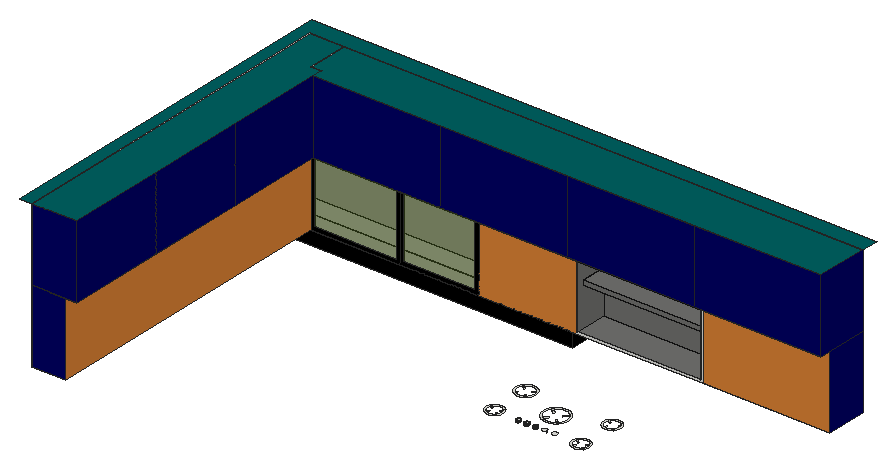
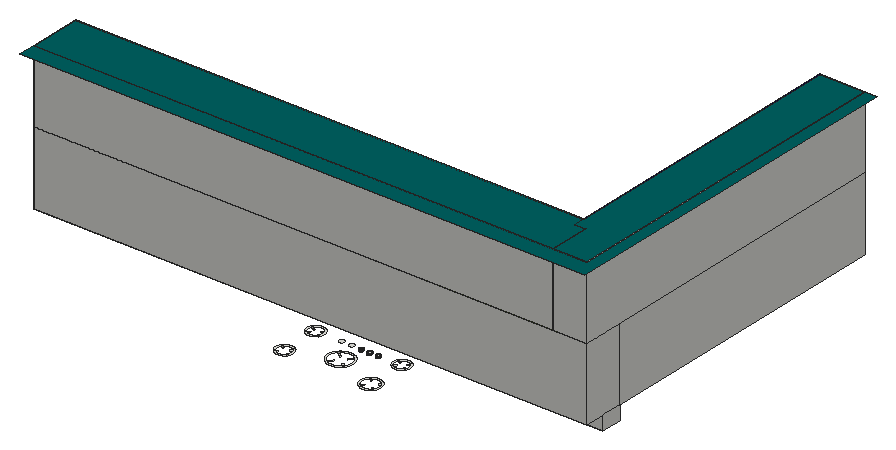
# SketchUp Ruby script. Lengths in inches.
U = 1.inch
M = Sketchup.active_model
def pt(a) = Geom::Point3d.new(a.map { |v| v * U })
def face(e, loops, mat)
  f = e.add_face(loops[0].map { |a| pt(a) })
  loops[1..].each { |l| e.add_face(l.map { |a| pt(a) }).erase! }
  f.material = f.back_material = mat if mat
  f
end
# faces: each face lists its corners as indices into pts; further lists are holes
def faces(e, pts, list, mat = nil) = list.each { |f| face(e, (f[0].is_a?(Array) ? f : [f]).map { |l| l.map { |i| pts[i] } }, mat) }
# xy, xz, yz: faces in a plane at the given z, y or x. An outline is a flat list of corners, or four numbers for a rectangle; further outlines are holes
def ring(l) = l.size == 4 ? [[l[0], l[1]], [l[2], l[1]], [l[2], l[3]], [l[0], l[3]]] : l.each_slice(2).to_a
def flat(e, list, mat, &to3) = list.each { |f| face(e, (f[0].is_a?(Array) ? f : [f]).map { |l| ring(l).map { |u, v| to3.(u, v) } }, mat) }
def xy(e, z, list, mat = nil) = flat(e, list, mat) { |x, y| [x, y, z] }
def xz(e, y, list, mat = nil) = flat(e, list, mat) { |x, z| [x, y, z] }
def yz(e, x, list, mat = nil) = flat(e, list, mat) { |y, z| [x, y, z] }
def lines(e, pts, list) = list.each { |a, b| e.add_line(pt(pts[a]), pt(pts[b])) }
# prism: a flat outline (further loops are holes) pulled along v
def prism(e, loops, v, mat = nil)
  f = face(e, loops, mat); d = Geom::Vector3d.new(v.map { |x| x * U })
  f.pushpull(f.normal.samedirection?(d) ? d.length : -d.length)
end
def box(e, o, s, mat = nil) = prism(e, [[o, [o[0] + s[0], o[1], o[2]], [o[0] + s[0], o[1] + s[1], o[2]], [o[0], o[1] + s[1], o[2]]]], [0, 0, s[2]], mat)
def at(x, y, z, deg = 0) = Geom::Transformation.translation(pt([x, y, z])) * Geom::Transformation.rotation(ORIGIN, Z_AXIS, deg.degrees)
def axes(o, x, y, z) = Geom::Transformation.new([*x, 0, *y, 0, *z, 0, *pt(o).to_a, 1])
def part(name) = M.definitions.add(name)
# library, detail: a bought-in or finely detailed component or shape, given as its bounding box
def library(name, o, s) = part(name).tap { |d| box(d.entities, o, s) }
def detail(e, o, s) = box(e.add_group.entities, o, s)
def put(e, d, t, mat = nil) = e.add_instance(d, t).tap { |i| i.material = mat if mat }
def group(e, t, mat = nil) = e.add_group.tap { |g| g.transformation = t; g.material = mat if mat }.entities
root = M.entities
M.materials.add("[0079_Teal]").color = [0, 96, 96]
M.materials.add("[0105_Navy]").color = [0, 0, 99]
M.materials.add("[Color M09]").color = [0, 0, 0]
M.materials.add("[Translucent Glass Dark Green]").color = [50, 73, 4]
M.materials["[Translucent Glass Dark Green]"].alpha = 0.5
M.materials.add("[Translucent Glass Gray]").color = [0, 0, 0]
M.materials["[Translucent Glass Gray]"].alpha = 0.5
M.materials.add("[Wood Bamboo]").color = [219, 130, 53]
xy(root,254.3125,[[832.58,637.12,838.75,642.52,837.78,643.6,831.63,638.07],[859.45,639.53,860.47,641.1,853.45,645.15,852.51,643.53],[834.88,653.71,835.82,655.33,829.43,659.02,828.58,657.35],[852.77,654.76,859.45,660.59,858.27,662.05,851.61,656.05]])
xy(root,254.5,[[834.42,730.4,838.85,735.32,837.46,736.57,832.96,731.58],[858.27,732.91,859.45,734.36,854.32,738.09,853.22,736.57],[833.38,750.99,834.48,752.51,830.45,755.43,829.43,753.86],[854.32,752.51,858.27,756.89,856.94,758.22,852.93,753.76]])
xy(root,255.0625,[[722.22,684.24,731.81,694.89,729.65,696.84,720.06,686.1875,721.09,685.16],[758.29,685.16,760.34,687.22,749.23,697.28,747.14,694.89],[726.2,714.05,728.12,716.18,719.03,724.42,717.2,722.15],[749.23,714.24,759.31,725.44,758.29,726.47,757.16,727.39,757.05,727.28,747.07,716.18]])
xy(root,255.1875,[[647.3,727.57,649.04,728.98,643.57,734.45,641.99,732.875],[619.69,729.66,619.86,729.83,624.69,733.98,623.16,735.77,618.09,731.4375,618.79,730.5625],[645.15,751.5625,652.04,757.49,650.63,759.23,643.67,753.28],[623.16,751.71,624.74,753.28,618.79,759.23,617.38,757.49]])
xy(root,255.75,[[622.85,637.29,629.08,642.73,627.88,644.1,621.58,638.6],[649.15,640.36,649.66,641.12,650.09,641.92,643.42,645.67,642.53,644.09],[624.89,654.02,625.78,655.61,619.76,659,618.91,657.39],[642.65,654.57,648.96,660.08,647.84,661.51,641.46,655.95]])
xy(root,256.875,[[[844.95,629.31,847.12,629.42,849.27,629.76,851.36,630.32,853.39,631.1,855.33,632.09,857.15,633.27,858.84,634.64,860.37,636.17,861.74,637.86,862.92,639.68,863.91,641.62,864.6875,643.65,865.25,645.74,865.59,647.89,865.7,650.06,865.59,652.23,865.25,654.375,864.6875,656.47,863.91,658.5,862.92,660.43,861.74,662.26,860.37,663.94,858.84,665.48,857.15,666.85,855.33,668.03,853.39,669.02,851.36,669.79,849.27,670.36,847.12,670.7,844.95,670.81,842.78,670.7,840.64,670.36,838.54,669.79,836.51,669.02,834.58,668.03,832.76,666.85,831.07,665.48,829.53,663.94,828.16,662.26,826.98,660.43,826,658.5,825.22,656.47,824.66,654.375,824.32,652.23,824.2,650.06,824.32,647.89,824.66,645.74,825.22,643.65,826,641.62,826.98,639.68,828.16,637.86,829.53,636.17,831.07,634.64,832.76,633.27,834.58,632.09,836.51,631.1,838.54,630.32,840.64,629.76,842.78,629.42],[844.95,632.14,843.08,632.24,841.23,632.53,839.41,633.01,837.66,633.6875,835.99,634.54,834.42,635.56,832.96,636.74,831.63,638.07,830.45,639.53,829.43,641.1,828.58,642.77,827.91,644.52,827.42,646.33,827.13,648.1875,827.03,650.06,827.13,651.93,827.42,653.79,827.91,655.6,828.58,657.35,829.43,659.02,830.45,660.59,831.63,662.05,832.96,663.38,834.42,664.56,835.99,665.58,837.66,666.43,839.41,667.1,841.23,667.59,843.08,667.88,844.95,667.98,846.82,667.88,848.68,667.59,850.49,667.1,852.24,666.43,853.91,665.58,855.49,664.56,856.94,663.38,858.27,662.05,859.45,660.59,860.47,659.02,861.32,657.35,862,655.6,862.48,653.79,862.77,651.93,862.875,650.06,862.77,648.1875,862.48,646.33,862,644.52,861.32,642.77,860.47,641.1,859.45,639.53,858.27,638.07,856.94,636.74,855.49,635.56,853.91,634.54,852.24,633.6875,850.49,633.01,848.68,632.53,846.82,632.24]],[[634.4,629.8125,636.51,629.89,638.61,630.1875,640.67,630.71,642.66,631.43,644.5625,632.37,646.36,633.49,648.02,634.8,649.55,636.28,650.91,637.9,652.09,639.66,653.08,641.54,653.87,643.5,654.45,645.54,654.8125,647.63,654.96,649.74,654.88,651.86,654.58,653.96,654.0625,656.02,653.33,658.01,652.4,659.91,651.28,661.71,649.97,663.375,648.49,664.9,646.87,666.25,645.11,667.4375,643.23,668.43,641.27,669.22,639.23,669.8,637.14,670.16,635.02,670.31,632.91,670.23,630.81,669.93,628.75,669.41,626.76,668.68,624.86,667.75,623.0625,666.625,621.4,665.32,619.875,663.84,618.51,662.21,617.33,660.45,616.34,658.58,615.55,656.61,614.97,654.58,614.61,652.49,614.46,650.375,614.54,648.26,614.84,646.16,615.36,644.1,616.08,642.11,617.02,640.21,618.14,638.41,619.45,636.74,620.93,635.22,622.55,633.86,624.3125,632.68,626.1875,631.69,628.15,630.9,630.19,630.32,632.28,629.96],[634.4375,632.64,632.62,632.76,630.82,633.08,629.07,633.58,627.38,634.26,625.77,635.11,624.25,636.125,622.85,637.29,621.58,638.6,620.46,640.04,619.49,641.58,618.6875,643.22,618.06,644.93,617.61,646.7,617.36,648.51,617.29,650.33,617.41,652.15,617.73,653.95,618.23,655.7,618.91,657.39,619.76,659,620.78,660.52,621.95,661.92,623.25,663.19,624.69,664.31,626.23,665.28,627.87,666.08,629.58,666.71,631.35,667.15,633.16,667.41,634.98,667.48,636.8,667.35,638.6,667.04,640.35,666.54,642.04,665.86,643.65,665.01,645.17,663.99,646.57,662.82,647.84,661.51,648.96,660.08,649.93,658.53,650.73,656.9,651.36,655.18,651.8,653.42,652.0625,651.61,652.13,649.79,652.01,647.97,651.69,646.17,651.19,644.42,650.51,642.73,649.66,641.12,648.64,639.6,647.47,638.2,646.16,636.93,644.73,635.81,643.19,634.84,641.55,634.04,639.84,633.41,638.07,632.96,636.26,632.71]],[713.34,644.32,713.91,644.35,714.47,644.4375,715.02,644.58,715.55,644.79,716.06,645.05,716.53,645.36,716.98,645.71,717.38,646.12,717.74,646.56,718.05,647.04,718.31,647.54,718.51,648.07,718.66,648.625,718.75,649.1875,718.78,649.75,718.75,650.32,718.66,650.89,718.51,651.43,718.31,651.97,718.05,652.47,717.74,652.95,717.38,653.39,716.98,653.8,716.53,654.15,716.06,654.46,715.55,654.72,715.02,654.93,714.47,655.07,713.91,655.16,713.34,655.19,712.77,655.16,712.21,655.07,711.66,654.93,711.125,654.72,710.62,654.46,710.14,654.15,709.7,653.8,709.3,653.39,708.9375,652.95,708.63,652.47,708.37,651.97,708.17,651.43,708.02,650.89,707.93,650.32,707.9,649.75,707.93,649.1875,708.02,648.625,708.17,648.07,708.37,647.54,708.63,647.04,708.9375,646.56,709.3,646.12,709.7,645.71,710.14,645.36,710.62,645.05,711.125,644.79,711.66,644.58,712.21,644.4375,712.77,644.35],[781.2,644.44,781.76,644.47,782.31,644.56,782.85,644.7,783.36,644.9,783.86,645.15,784.33,645.46,784.76,645.81,785.15,646.2,785.5,646.63,785.8,647.1,786.06,647.59,786.26,648.11,786.4,648.65,786.49,649.2,786.52,649.75,786.49,650.31,786.4,650.86,786.26,651.4,786.06,651.92,785.8,652.41,785.5,652.88,785.15,653.31,784.76,653.7,784.33,654.05,783.86,654.36,783.36,654.61,782.85,654.81,782.31,654.95,781.76,655.04,781.2,655.07,780.65,655.04,780.1,654.95,779.5625,654.81,779.04,654.61,778.55,654.36,778.08,654.05,777.65,653.7,777.26,653.31,776.91,652.88,776.6,652.41,776.35,651.92,776.15,651.4,776.01,650.86,775.92,650.31,775.89,649.75,775.92,649.2,776.01,648.65,776.15,648.11,776.35,647.59,776.6,647.1,776.91,646.63,777.26,646.2,777.65,645.81,778.08,645.46,778.55,645.15,779.04,644.9,779.5625,644.7,780.1,644.56,780.65,644.47],[756.84,644.69,757.37,644.72,757.89,644.8,758.4,644.94,758.9,645.13,759.37,645.37,759.82,645.66,760.23,645.99,760.6,646.37,760.94,646.78,761.22,647.22,761.46,647.7,761.65,648.19,761.79,648.7,761.875,649.23,761.9,649.75,761.875,650.28,761.79,650.81,761.65,651.32,761.46,651.8125,761.22,652.29,760.94,652.73,760.6,653.14,760.23,653.52,759.82,653.85,759.37,654.14,758.9,654.38,758.4,654.57,757.89,654.71,757.37,654.79,756.84,654.82,756.3125,654.79,755.79,654.71,755.28,654.57,754.78,654.38,754.31,654.14,753.86,653.85,753.45,653.52,753.08,653.14,752.74,652.73,752.46,652.29,752.21,651.8125,752.02,651.32,751.89,650.81,751.8,650.28,751.78,649.75,751.8,649.23,751.89,648.7,752.02,648.19,752.21,647.7,752.46,647.22,752.74,646.78,753.08,646.37,753.45,645.99,753.86,645.66,754.31,645.37,754.78,645.13,755.28,644.94,755.79,644.8,756.3125,644.72],
  [734.71,644.78,735.23,644.81,735.75,644.89,736.25,645.03,736.74,645.21,737.2,645.45,737.64,645.73,738.04,646.06,738.41,646.43,738.74,646.83,739.02,647.27,739.26,647.73,739.44,648.22,739.58,648.72,739.66,649.23,739.6875,649.75,739.66,650.27,739.58,650.79,739.44,651.29,739.26,651.78,739.02,652.24,738.74,652.68,738.41,653.08,738.04,653.45,737.64,653.78,737.2,654.0625,736.74,654.3,736.25,654.48,735.75,654.62,735.23,654.7,734.71,654.73,734.19,654.7,733.68,654.62,733.18,654.48,732.69,654.3,732.23,654.0625,731.79,653.78,731.39,653.45,731.02,653.08,730.69,652.68,730.41,652.24,730.17,651.78,729.98,651.29,729.85,650.79,729.77,650.27,729.74,649.75,729.77,649.23,729.85,648.72,729.98,648.22,730.17,647.73,730.41,647.27,730.69,646.83,731.02,646.43,731.39,646.06,731.79,645.73,732.23,645.45,732.69,645.21,733.18,645.03,733.68,644.89,734.19,644.81],[693.15,644.94,693.65,644.97,694.15,645.05,694.63,645.18,695.1,645.36,695.55,645.59,695.97,645.86,696.37,646.18,696.72,646.53,697.04,646.93,697.3125,647.35,697.54,647.8,697.72,648.27,697.85,648.75,697.93,649.25,697.96,649.75,697.93,650.26,697.85,650.76,697.72,651.24,697.54,651.71,697.3125,652.16,697.04,652.58,696.72,652.97,696.37,653.33,695.97,653.65,695.55,653.92,695.1,654.15,694.63,654.33,694.15,654.46,693.65,654.54,693.15,654.57,692.64,654.54,692.14,654.46,691.66,654.33,691.1875,654.15,690.74,653.92,690.32,653.65,689.93,653.33,689.57,652.97,689.25,652.58,688.98,652.16,688.75,651.71,688.57,651.24,688.4375,650.76,688.36,650.26,688.33,649.75,688.36,649.25,688.4375,648.75,688.57,648.27,688.75,647.8,688.98,647.35,689.25,646.93,689.57,646.53,689.93,646.18,690.32,645.86,690.74,645.59,691.1875,645.36,691.66,645.18,692.14,645.05,692.64,644.97],[[739.6875,675.19,742.89,675.36,746.05,675.86,749.15,676.69,752.14,677.84,755,679.29,757.6875,681.04,760.18,683.06,762.45,685.32,764.46,687.82,766.21,690.5,767.66,693.36,768.8125,696.35,769.64,699.45,770.14,702.61,770.3125,705.82,770.14,709.02,769.64,712.18,768.8125,715.28,767.66,718.27,766.21,721.13,764.46,723.82,762.45,726.31,760.18,728.57,757.6875,730.59,755,732.34,752.14,733.79,749.15,734.94,746.05,735.77,742.89,736.27,739.6875,736.44,736.49,736.27,733.32,735.77,730.22,734.94,727.23,733.79,724.375,732.34,721.6875,730.59,719.19,728.57,716.93,726.31,714.91,723.82,713.16,721.13,711.71,718.27,710.5625,715.28,709.73,712.18,709.23,709.02,709.0625,705.82,709.23,702.61,709.73,699.45,710.5625,696.35,711.71,693.36,713.16,690.5,714.91,687.82,716.93,685.32,719.19,683.06,721.6875,681.04,724.375,679.29,727.23,677.84,730.22,676.69,733.32,675.86,736.49,675.36],[739.6875,678.02,736.78,678.17,733.91,678.625,731.1,679.38,728.38,680.42,725.79,681.74,723.35,683.33,721.09,685.16,719.03,687.22,717.2,689.48,715.61,691.92,714.29,694.51,713.25,697.23,712.5,700.04,712.04,702.91,711.89,705.82,712.04,708.72,712.5,711.6,713.25,714.41,714.29,717.12,715.61,719.71,717.2,722.15,719.03,724.42,721.09,726.47,723.35,728.3,725.79,729.89,728.38,731.21,731.1,732.25,733.91,733,736.78,733.46,739.6875,733.61,742.59,733.46,745.47,733,748.28,732.25,750.99,731.21,753.58,729.89,756.03,728.3,758.29,726.47,760.34,724.42,762.17,722.15,763.76,719.71,765.08,717.12,766.12,714.41,766.875,711.6,767.33,708.72,767.48,705.82,767.33,702.91,766.875,700.04,766.12,697.23,765.08,694.51,763.76,691.92,762.17,689.48,760.34,687.22,758.29,685.16,756.03,683.33,753.58,681.74,750.99,680.42,748.28,679.38,745.47,678.625,742.59,678.17]],[[634.71,720.65,637.24,720.78,639.75,721.18,642.2,721.84,644.57,722.74,646.83,723.9,648.96,725.28,650.9375,726.875,652.73,728.67,654.33,730.64,655.71,732.77,656.86,735.03,657.77,737.4,658.43,739.86,658.83,742.36,658.96,744.9,658.83,747.43,658.43,749.94,657.77,752.39,656.86,754.76,655.71,757.02,654.33,759.15,652.73,761.125,650.9375,762.92,648.96,764.52,646.83,765.9,644.57,767.05,642.2,767.96,639.75,768.62,637.24,769.02,634.71,769.15,632.18,769.02,629.67,768.62,627.22,767.96,624.85,767.05,622.58,765.9,620.46,764.52,618.48,762.92,616.6875,761.125,615.09,759.15,613.71,757.02,612.56,754.76,611.65,752.39,610.99,749.94,610.59,747.43,610.46,744.9,610.59,742.36,610.99,739.86,611.65,737.4,612.56,735.03,613.71,732.77,615.09,730.64,616.6875,728.67,618.48,726.875,620.46,725.28,622.58,723.9,624.85,722.74,627.22,721.84,629.67,721.18,632.18,720.78],[634.71,723.48,632.47,723.59,630.26,723.94,628.09,724.53,626,725.33,624,726.35,622.12,727.57,620.375,728.98,618.79,730.5625,617.38,732.31,616.16,734.1875,615.14,736.19,614.34,738.28,613.76,740.44,613.41,742.66,613.29,744.9,613.41,747.14,613.76,749.35,614.34,751.52,615.14,753.61,616.16,755.61,617.38,757.49,618.79,759.23,620.375,760.82,622.12,762.23,624,763.45,626,764.47,628.09,765.27,630.26,765.85,632.47,766.2,634.71,766.32,636.95,766.2,639.16,765.85,641.33,765.27,643.42,764.47,645.42,763.45,647.3,762.23,649.04,760.82,650.63,759.23,652.04,757.49,653.26,755.61,654.28,753.61,655.08,751.52,655.66,749.35,656.01,747.14,656.13,744.9,656.01,742.66,655.66,740.44,655.08,738.28,654.28,736.19,653.26,734.1875,652.04,732.31,650.63,730.5625,649.04,728.98,647.3,727.57,645.42,726.35,643.42,725.33,641.33,724.53,639.16,723.94,636.95,723.59]],[[844.95,724.15,847.12,724.26,849.27,724.6,851.36,725.16,853.39,725.94,855.33,726.93,857.15,728.11,858.84,729.48,860.37,731.01,861.74,732.7,862.92,734.52,863.91,736.46,864.6875,738.49,865.25,740.58,865.59,742.73,865.7,744.9,865.59,747.07,865.25,749.21,864.6875,751.31,863.91,753.34,862.92,755.27,861.74,757.09,860.37,758.78,858.84,760.32,857.15,761.69,855.33,762.87,853.39,763.85,851.36,764.63,849.27,765.19,847.12,765.53,844.95,765.65,842.78,765.53,840.64,765.19,838.54,764.63,836.51,763.85,834.58,762.87,832.76,761.69,831.07,760.32,829.53,758.78,828.16,757.09,826.98,755.27,826,753.34,825.22,751.31,824.66,749.21,824.32,747.07,824.2,744.9,824.32,742.73,824.66,740.58,825.22,738.49,826,736.46,826.98,734.52,828.16,732.7,829.53,731.01,831.07,729.48,832.76,728.11,834.58,726.93,836.51,725.94,838.54,725.16,840.64,724.6,842.78,724.26],[844.95,726.98,843.08,727.07,841.23,727.37,839.41,727.85,837.66,728.53,835.99,729.38,834.42,730.4,832.96,731.58,831.63,732.91,830.45,734.36,829.43,735.9375,828.58,737.61,827.91,739.36,827.42,741.17,827.13,743.02,827.03,744.9,827.13,746.77,827.42,748.625,827.91,750.4375,828.58,752.1875,829.43,753.86,830.45,755.43,831.63,756.89,832.96,758.22,834.42,759.4,835.99,760.42,837.66,761.27,839.41,761.94,841.23,762.43,843.08,762.72,844.95,762.82,846.82,762.72,848.68,762.43,850.49,761.94,852.24,761.27,853.91,760.42,855.49,759.4,856.94,758.22,858.27,756.89,859.45,755.43,860.47,753.86,861.32,752.1875,862,750.4375,862.48,748.625,862.77,746.77,862.875,744.9,862.77,743.02,862.48,741.17,862,739.36,861.32,737.61,860.47,735.9375,859.45,734.36,858.27,732.91,856.94,731.58,855.49,730.4,853.91,729.38,852.24,728.53,850.49,727.85,848.68,727.37,846.82,727.07]]])
xy(root,390.15,[[28.58,745.5625,747.58,795.66]],"[Color M09]")
xy(root,424.15,[[28.58,745.5625,747.58,795.66],[747.58,745.5625,747.58,795.66,28.58,795.66,28.58,845.75,1373.86,845.75,1373.86,745.5625]])
xy(root,424.15,[[28.58,0,111.52,745.5625]],"[Color M09]")
xy(root,429.67,[[761.09,745.5625,1059.19,822.875]])
xy(root,525,[[761.09,760.375,1059.19,822.875]])
xy(root,536.49,[[761.09,760.375,1059.19,822.875]])
xy(root,596.46,[[761.09,745.5625,1059.19,822.875]])
xy(root,601.98,[[28.58,0,111.52,745.5625],[28.58,745.5625,111.52,845.75],[111.52,745.5625,1373.86,845.75]])
xy(root,601.98,[[111.52,0,111.52,745.5625,1373.86,745.5625,1373.86,719.8125,137.27,719.8125,137.27,0]],"[Wood Bamboo]")
xy(root,779.8125,[[0,0,28.58,0,28.58,845.75,1373.86,845.75,1373.86,887.375,0,887.375],[28.58,0,137.27,0,137.27,745.5625,111.52,745.5625,111.52,845.75,28.58,845.75],[137.27,719.8125,1373.86,719.8125,1373.86,845.75,111.52,845.75,111.52,745.5625,137.27,745.5625]],"[0079_Teal]")
xz(root,0,[[28.58,424.15,111.52,601.98],[28.58,601.98,137.27,779.8125]],"[0105_Navy]")
xz(root,719.8125,[[137.27,601.98,446.42,779.8125],[446.42,601.98,755.57,779.8125],[755.57,601.98,1064.72,779.8125],[1064.72,601.98,1373.86,779.8125]],"[0105_Navy]")
xz(root,745.5625,[[28.58,424.15,111.52,601.98],[[755.57,424.15,1064.72,601.98],[761.09,429.67,1059.19,596.46]],[111.52,601.98,137.27,779.8125]])
xz(root,745.5625,[[28.58,390.15,747.58,424.15],[[111.52,424.15,328.1875,601.98],[119.9,432.53,319.81,593.6]],[[328.1875,424.15,519.1,601.98],[336.57,432.53,510.72,593.6]]],"[Color M09]")
xz(root,745.5625,[[119.9,432.53,319.81,593.6],[336.57,432.53,510.72,593.6]],"[Translucent Glass Dark Green]")
xz(root,745.5625,[[761.09,429.67,1059.19,596.46]],"[Translucent Glass Gray]")
xz(root,745.5625,[[519.1,424.15,755.57,601.98],[1064.72,424.15,1373.86,601.98]],"[Wood Bamboo]")
xz(root,760.375,[[761.09,525,1059.19,536.49]])
xz(root,795.66,[[28.58,390.15,747.58,424.15]])
xz(root,822.875,[[761.09,429.67,1059.19,525],[761.09,525,1059.19,536.49],[761.09,536.49,1059.19,596.46]])
xz(root,845.75,[[28.58,424.15,1373.86,601.98],[28.58,601.98,111.52,779.8125],[111.52,601.98,1373.86,779.8125]])
yz(root,28.58,[[745.5625,390.15,795.66,424.15],[0,424.15,745.5625,601.98],[745.5625,424.15,845.75,601.98],[0,601.98,845.75,779.8125]])
yz(root,111.52,[[745.5625,601.98,845.75,779.8125]])
yz(root,111.52,[[0,424.15,745.5625,601.98]],"[Wood Bamboo]")
yz(root,137.27,[[0,601.98,239.9375,779.8125],[239.9375,601.98,479.875,779.8125],[479.875,601.98,719.8125,779.8125]],"[0105_Navy]")
yz(root,747.58,[[745.5625,390.15,795.66,424.15]],"[Color M09]")
yz(root,761.09,[[745.5625,429.67,822.875,429.67,822.875,525,760.375,525,760.375,536.49,822.875,536.49,822.875,596.46,745.5625,596.46],[760.375,525,822.875,536.49]])
yz(root,1059.19,[[745.5625,429.67,745.5625,596.46,822.875,596.46,822.875,536.49,760.375,536.49,760.375,525,822.875,525,822.875,429.67],[760.375,525,822.875,536.49]])
yz(root,1373.86,[[745.5625,424.15,845.75,601.98],[719.8125,601.98,845.75,779.8125]],"[0105_Navy]")
p = [[712.21,644.4375,253.1875],[712.77,644.35,253.1875],[712.77,644.35,256.875],[712.21,644.4375,256.875],[713.34,644.32,253.1875],[713.34,644.32,256.875],
  [713.91,644.35,253.1875],[713.91,644.35,256.875],[714.47,644.4375,253.1875],[714.47,644.4375,256.875],[711.66,644.58,253.1875],[711.66,644.58,256.875],
  [715.02,644.58,253.1875],[715.02,644.58,256.875],[711.125,644.79,253.1875],[711.125,644.79,256.875],[715.55,644.79,253.1875],[715.55,644.79,256.875],
  [710.62,645.05,253.1875],[710.62,645.05,256.875],[716.06,645.05,253.1875],[716.06,645.05,256.875],[733.68,644.89,253.1875],[734.19,644.81,253.1875],
  [734.19,644.81,256.875],[733.68,644.89,256.875],[734.71,644.78,253.1875],[734.71,644.78,256.875],[735.23,644.81,253.1875],[735.23,644.81,256.875],
  [735.75,644.89,253.1875],[735.75,644.89,256.875],[692.64,644.97,253.1875],[693.15,644.94,253.1875],[693.15,644.94,256.875],[692.64,644.97,256.875],
  [693.65,644.97,253.1875],[693.65,644.97,256.875],[733.18,645.03,253.1875],[733.18,645.03,256.875],[736.25,645.03,253.1875],[736.25,645.03,256.875],
  [691.66,645.18,253.1875],[692.14,645.05,253.1875],[692.14,645.05,256.875],[691.66,645.18,256.875],[694.15,645.05,253.1875],[694.15,645.05,256.875],
  [694.63,645.18,253.1875],[694.63,645.18,256.875],[710.14,645.36,253.1875],[710.14,645.36,256.875],[716.53,645.36,253.1875],[716.53,645.36,256.875],
  [732.69,645.21,253.1875],[732.69,645.21,256.875],[736.74,645.21,253.1875],[736.74,645.21,256.875],[691.1875,645.36,253.1875],[691.1875,645.36,256.875],
  [695.1,645.36,253.1875],[695.1,645.36,256.875],[732.23,645.45,253.1875],[732.23,645.45,256.875],[737.2,645.45,253.1875],[737.2,645.45,256.875],
  [690.74,645.59,253.1875],[690.74,645.59,256.875],[695.55,645.59,253.1875],[695.55,645.59,256.875],[709.7,645.71,253.1875],[709.7,645.71,256.875],
  [716.98,645.71,253.1875],[716.98,645.71,256.875],[731.79,645.73,253.1875],[731.79,645.73,256.875],[737.64,645.73,253.1875],[737.64,645.73,256.875],
  [690.32,645.86,253.1875],[690.32,645.86,256.875],[695.97,645.86,253.1875],[695.97,645.86,256.875],[709.3,646.12,253.1875],[709.3,646.12,256.875],
  [717.38,646.12,253.1875],[717.38,646.12,256.875],[731.39,646.06,253.1875],[731.39,646.06,256.875],[738.04,646.06,253.1875],[738.04,646.06,256.875],
  [689.93,646.18,253.1875],[689.93,646.18,256.875],[696.37,646.18,253.1875],[696.37,646.18,256.875],[708.9375,646.56,253.1875],[708.9375,646.56,256.875],
  [717.74,646.56,253.1875],[717.74,646.56,256.875],[731.02,646.43,253.1875],[731.02,646.43,256.875],[738.41,646.43,253.1875],[738.41,646.43,256.875],
  [689.57,646.53,253.1875],[689.57,646.53,256.875],[696.72,646.53,253.1875],[696.72,646.53,256.875],[730.69,646.83,253.1875],[730.69,646.83,256.875],
  [738.74,646.83,253.1875],[738.74,646.83,256.875],[689.25,646.93,253.1875],[689.25,646.93,256.875],[697.04,646.93,253.1875],[697.04,646.93,256.875],
  [708.63,647.04,253.1875],[708.63,647.04,256.875],[718.05,647.04,253.1875],[718.05,647.04,256.875],[730.41,647.27,253.1875],[730.41,647.27,256.875],
  [739.02,647.27,253.1875],[739.02,647.27,256.875],[688.98,647.35,253.1875],[688.98,647.35,256.875],[697.3125,647.35,253.1875],[697.3125,647.35,256.875],
  [708.37,647.54,253.1875],[708.37,647.54,256.875],[718.31,647.54,253.1875],[718.31,647.54,256.875],[688.75,647.8,253.1875],[688.75,647.8,256.875],
  [697.54,647.8,253.1875],[697.54,647.8,256.875],[730.17,647.73,253.1875],[730.17,647.73,256.875],[739.26,647.73,253.1875],[739.26,647.73,256.875],
  [708.17,648.07,253.1875],[708.17,648.07,256.875],[718.51,648.07,253.1875],[718.51,648.07,256.875],[729.98,648.22,253.1875],[729.98,648.22,256.875],
  [739.44,648.22,253.1875],[739.44,648.22,256.875],[688.57,648.27,253.1875],[688.57,648.27,256.875],[697.72,648.27,253.1875],[697.72,648.27,256.875],
  [708.02,648.625,253.1875],[708.02,648.625,256.875],[718.66,648.625,253.1875],[718.66,648.625,256.875],[729.85,648.72,253.1875],[729.85,648.72,256.875],
  [739.58,648.72,253.1875],[739.58,648.72,256.875],[688.4375,648.75,253.1875],[688.4375,648.75,256.875],[697.85,648.75,253.1875],[697.85,648.75,256.875],
  [707.93,649.1875,253.1875],[707.93,649.1875,256.875],[718.75,649.1875,253.1875],[718.75,649.1875,256.875],[729.77,649.23,253.1875],[729.77,649.23,256.875],
  [739.66,649.23,253.1875],[739.66,649.23,256.875],[761.79,648.7,253.1875],[761.875,649.23,253.1875],[761.875,649.23,256.875],[761.79,648.7,256.875],
  [688.36,649.25,253.1875],[688.36,649.25,256.875],[697.93,649.25,253.1875],[697.93,649.25,256.875],[707.9,649.75,253.1875],[707.9,649.75,256.875],
  [718.78,649.75,253.1875],[718.78,649.75,256.875],[729.74,649.75,253.1875],[729.74,649.75,256.875],[739.6875,649.75,253.1875],[739.6875,649.75,256.875],
  [761.9,649.75,253.1875],[761.9,649.75,256.875],[688.33,649.75,253.1875],[688.33,649.75,256.875],[697.96,649.75,253.1875],[697.96,649.75,256.875],
  [688.36,650.26,253.1875],[688.36,650.26,256.875],[697.93,650.26,253.1875],[697.93,650.26,256.875],[707.93,650.32,253.1875],[707.93,650.32,256.875],
  [718.75,650.32,253.1875],[718.75,650.32,256.875],[729.77,650.27,253.1875],[729.77,650.27,256.875],[739.66,650.27,253.1875],[739.66,650.27,256.875],
  [688.4375,650.76,253.1875],[688.4375,650.76,256.875],[697.85,650.76,253.1875],[697.85,650.76,256.875],[708.02,650.89,253.1875],[708.02,650.89,256.875],
  [718.66,650.89,253.1875],[718.66,650.89,256.875],[729.85,650.79,253.1875],[729.85,650.79,256.875],[739.58,650.79,253.1875],[739.58,650.79,256.875],
  [688.57,651.24,253.1875],[688.57,651.24,256.875],[697.72,651.24,253.1875],[697.72,651.24,256.875],[729.98,651.29,253.1875],[729.98,651.29,256.875],
  [739.44,651.29,253.1875],[739.44,651.29,256.875],[708.17,651.43,253.1875],[708.17,651.43,256.875],[718.51,651.43,253.1875],[718.51,651.43,256.875],
  [688.75,651.71,253.1875],[688.75,651.71,256.875],[697.54,651.71,253.1875],[697.54,651.71,256.875],[730.17,651.78,253.1875],[730.17,651.78,256.875],
  [739.26,651.78,253.1875],[739.26,651.78,256.875],[708.37,651.97,253.1875],[708.37,651.97,256.875],[718.31,651.97,253.1875],[718.31,651.97,256.875],
  [688.98,652.16,253.1875],[688.98,652.16,256.875],[697.3125,652.16,253.1875],[697.3125,652.16,256.875],[730.41,652.24,253.1875],[730.41,652.24,256.875],
  [739.02,652.24,253.1875],[739.02,652.24,256.875],[708.63,652.47,253.1875],[708.63,652.47,256.875],[718.05,652.47,253.1875],[718.05,652.47,256.875],
  [689.25,652.58,253.1875],[689.25,652.58,256.875],[697.04,652.58,253.1875],[697.04,652.58,256.875],[730.69,652.68,253.1875],[730.69,652.68,256.875],
  [738.74,652.68,253.1875],[738.74,652.68,256.875],[708.9375,652.95,253.1875],[708.9375,652.95,256.875],[717.74,652.95,253.1875],[717.74,652.95,256.875],
  [689.57,652.97,253.1875],[689.57,652.97,256.875],[696.72,652.97,253.1875],[696.72,652.97,256.875],[731.02,653.08,253.1875],[731.02,653.08,256.875],
  [738.41,653.08,253.1875],[738.41,653.08,256.875],[689.93,653.33,253.1875],[689.93,653.33,256.875],[696.37,653.33,253.1875],[696.37,653.33,256.875],
  [709.3,653.39,253.1875],[709.3,653.39,256.875],[717.38,653.39,253.1875],[717.38,653.39,256.875],[731.39,653.45,253.1875],[731.39,653.45,256.875],
  [738.04,653.45,253.1875],[738.04,653.45,256.875],[690.32,653.65,253.1875],[690.32,653.65,256.875],[695.97,653.65,253.1875],[695.97,653.65,256.875],
  [709.7,653.8,253.1875],[709.7,653.8,256.875],[716.98,653.8,253.1875],[716.98,653.8,256.875],[731.79,653.78,253.1875],[731.79,653.78,256.875],
  [737.64,653.78,253.1875],[737.64,653.78,256.875],[690.74,653.92,253.1875],[690.74,653.92,256.875],[695.55,653.92,253.1875],[695.55,653.92,256.875],
  [710.14,654.15,253.1875],[710.14,654.15,256.875],[716.53,654.15,253.1875],[716.53,654.15,256.875],[732.23,654.0625,253.1875],[732.23,654.0625,256.875],
  [737.2,654.0625,253.1875],[737.2,654.0625,256.875],[691.1875,654.15,253.1875],[691.1875,654.15,256.875],[695.1,654.15,253.1875],[695.1,654.15,256.875],
  [732.69,654.3,253.1875],[732.69,654.3,256.875],[736.74,654.3,253.1875],[736.74,654.3,256.875],[691.66,654.33,253.1875],[691.66,654.33,256.875],
  [694.63,654.33,253.1875],[694.63,654.33,256.875],[710.62,654.46,253.1875],[710.62,654.46,256.875],[716.06,654.46,253.1875],[716.06,654.46,256.875],
  [692.14,654.46,253.1875],[692.14,654.46,256.875],[694.15,654.46,253.1875],[694.15,654.46,256.875],[733.18,654.48,253.1875],[733.18,654.48,256.875],
  [736.25,654.48,253.1875],[736.25,654.48,256.875],[692.64,654.54,253.1875],[692.64,654.54,256.875],[693.15,654.57,253.1875],[693.15,654.57,256.875],
  [693.65,654.54,253.1875],[693.65,654.54,256.875],[711.125,654.72,253.1875],[711.125,654.72,256.875],[715.55,654.72,253.1875],[715.55,654.72,256.875],
  [733.68,654.62,253.1875],[733.68,654.62,256.875],[735.75,654.62,253.1875],[735.75,654.62,256.875],[734.19,654.7,253.1875],[734.19,654.7,256.875],
  [735.23,654.7,253.1875],[735.23,654.7,256.875],[711.66,654.93,253.1875],[711.66,654.93,256.875],[715.02,654.93,253.1875],[715.02,654.93,256.875],
  [734.71,654.73,253.1875],[734.71,654.73,256.875],[712.21,655.07,253.1875],[712.21,655.07,256.875],[714.47,655.07,253.1875],[714.47,655.07,256.875],
  [712.77,655.16,253.1875],[712.77,655.16,256.875],[713.91,655.16,253.1875],[713.91,655.16,256.875],[713.34,655.19,253.1875],[713.34,655.19,256.875],
  [860.47,641.1,256.875],[860.47,641.1,254.3125],[859.45,639.53,254.3125],[859.45,639.53,256.875],[828.58,657.35,256.875],[828.58,657.35,254.3125],
  [829.43,659.02,254.3125],[829.43,659.02,256.875],[858.27,662.05,256.875],[858.27,662.05,254.3125],[859.45,660.59,254.3125],[859.45,660.59,256.875],
  [834.42,730.4,256.875],[834.42,730.4,254.5],[832.96,731.58,254.5],[832.96,731.58,256.875],[859.45,734.36,256.875],[859.45,734.36,254.5],
  [858.27,732.91,254.5],[858.27,732.91,256.875],[829.43,753.86,256.875],[829.43,753.86,254.5],[830.45,755.43,254.5],[830.45,755.43,256.875],
  [856.94,758.22,256.875],[856.94,758.22,254.5],[858.27,756.89,254.5],[858.27,756.89,256.875],[760.34,687.22,256.875],[760.34,687.22,255.0625],
  [758.29,685.16,255.0625],[758.29,685.16,256.875],[717.2,722.15,256.875],[717.2,722.15,255.0625],[719.03,724.42,255.0625],[719.03,724.42,256.875],
  [649.04,728.98,256.875],[649.04,728.98,255.1875],[647.3,727.57,255.1875],[647.3,727.57,256.875],[617.38,757.49,256.875],[617.38,757.49,255.1875],
  [618.79,759.23,255.1875],[618.79,759.23,256.875],[650.63,759.23,256.875],[650.63,759.23,255.1875],[652.04,757.49,255.1875],[652.04,757.49,256.875],
  [622.85,637.29,256.875],[622.85,637.29,255.75],[621.58,638.6,255.75],[621.58,638.6,256.875],[618.91,657.39,256.875],[618.91,657.39,255.75],
  [619.76,659,255.75],[619.76,659,256.875],[647.84,661.51,256.875],[647.84,661.51,255.75],[648.96,660.08,255.75],[648.96,660.08,256.875]]
faces(root,p,[[0,1,2,3],[1,4,5,2],[4,6,7,5],[6,8,9,7],[10,0,3,11],[8,12,13,9],[14,10,11,15],[12,16,17,13],
  [18,14,15,19],[16,20,21,17],[22,23,24,25],[23,26,27,24],[26,28,29,27],[28,30,31,29],[32,33,34,35],[33,36,37,34],
  [38,22,25,39],[30,40,41,31],[42,43,44,45],[43,32,35,44],[36,46,47,37],[46,48,49,47],[50,18,19,51],[20,52,53,21],
  [54,38,39,55],[40,56,57,41],[58,42,45,59],[48,60,61,49],[62,54,55,63],[56,64,65,57],[66,58,59,67],[60,68,69,61],
  [70,50,51,71],[52,72,73,53],[74,62,63,75],[64,76,77,65],[78,66,67,79],[68,80,81,69],[82,70,71,83],[72,84,85,73],
  [86,74,75,87],[76,88,89,77],[90,78,79,91],[80,92,93,81],[94,82,83,95],[84,96,97,85],[98,86,87,99],[88,100,101,89],
  [102,90,91,103],[92,104,105,93],[106,98,99,107],[100,108,109,101],[110,102,103,111],[104,112,113,105],[114,94,95,115],[96,116,117,97],
  [118,106,107,119],[108,120,121,109],[122,110,111,123],[112,124,125,113],[126,114,115,127],[116,128,129,117],[130,122,123,131],[124,132,133,125],
  [134,118,119,135],[120,136,137,121],[138,126,127,139],[128,140,141,129],[142,134,135,143],[136,144,145,137],[146,130,131,147],[132,148,149,133],
  [150,138,139,151],[140,152,153,141],[154,142,143,155],[144,156,157,145],[158,146,147,159],[148,160,161,149],[162,150,151,163],[152,164,165,153],
  [166,154,155,167],[156,168,169,157],[170,171,172,173],[174,158,159,175],[160,176,177,161],[178,162,163,179],[164,180,181,165],[182,166,167,183],
  [168,184,185,169],[171,186,187,172],[188,174,175,189],[176,190,191,177],[192,188,189,193],[190,194,195,191],[196,178,179,197],[180,198,199,181],
  [200,182,183,201],[184,202,203,185],[204,192,193,205],[194,206,207,195],[208,196,197,209],[198,210,211,199],[212,200,201,213],[202,214,215,203],
  [216,204,205,217],[206,218,219,207],[220,212,213,221],[214,222,223,215],[224,208,209,225],[210,226,227,211],[228,216,217,229],[218,230,231,219],
  [232,220,221,233],[222,234,235,223],[236,224,225,237],[226,238,239,227],[240,228,229,241],[230,242,243,231],[244,232,233,245],[234,246,247,235],
  [248,236,237,249],[238,250,251,239],[252,240,241,253],[242,254,255,243],[256,244,245,257],[246,258,259,247],[260,248,249,261],[250,262,263,251],
  [264,252,253,265],[254,266,267,255],[268,256,257,269],[258,270,271,259],[272,264,265,273],[266,274,275,267],[276,260,261,277],[262,278,279,263],
  [280,268,269,281],[270,282,283,271],[284,272,273,285],[274,286,287,275],[288,276,277,289],[278,290,291,279],[292,280,281,293],[282,294,295,283],
  [296,284,285,297],[286,298,299,287],[300,288,289,301],[290,302,303,291],[304,292,293,305],[294,306,307,295],[308,296,297,309],[298,310,311,299],
  [312,304,305,313],[306,314,315,307],[316,308,309,317],[310,318,319,311],[320,300,301,321],[302,322,323,303],[324,316,317,325],[318,326,327,319],
  [328,312,313,329],[314,330,331,315],[332,324,325,333],[334,332,333,335],[336,334,335,337],[326,336,337,327],[338,320,321,339],[322,340,341,323],
  [342,328,329,343],[330,344,345,331],[346,342,343,347],[344,348,349,345],[350,338,339,351],[340,352,353,341],[354,346,347,355],[348,354,355,349],
  [356,350,351,357],[352,358,359,353],[360,356,357,361],[358,362,363,359],[364,360,361,365],[362,364,365,363],[366,367,368,369],[370,371,372,373],
  [374,375,376,377],[378,379,380,381],[382,383,384,385],[386,387,388,389],[390,391,392,393],[394,395,396,397],[398,399,400,401],[402,403,404,405],
  [406,407,408,409],[410,411,412,413],[414,415,416,417],[418,419,420,421],[422,423,424,425]])
